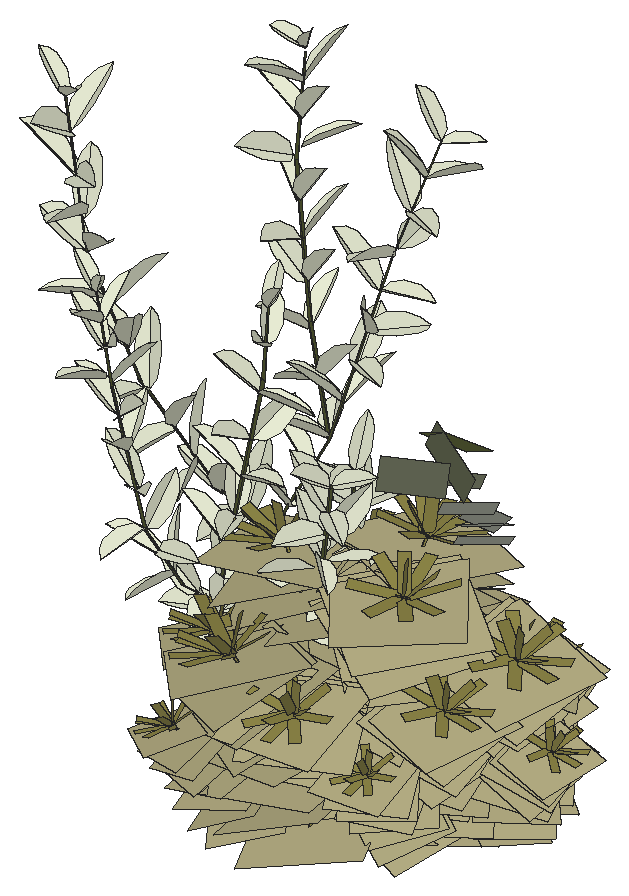
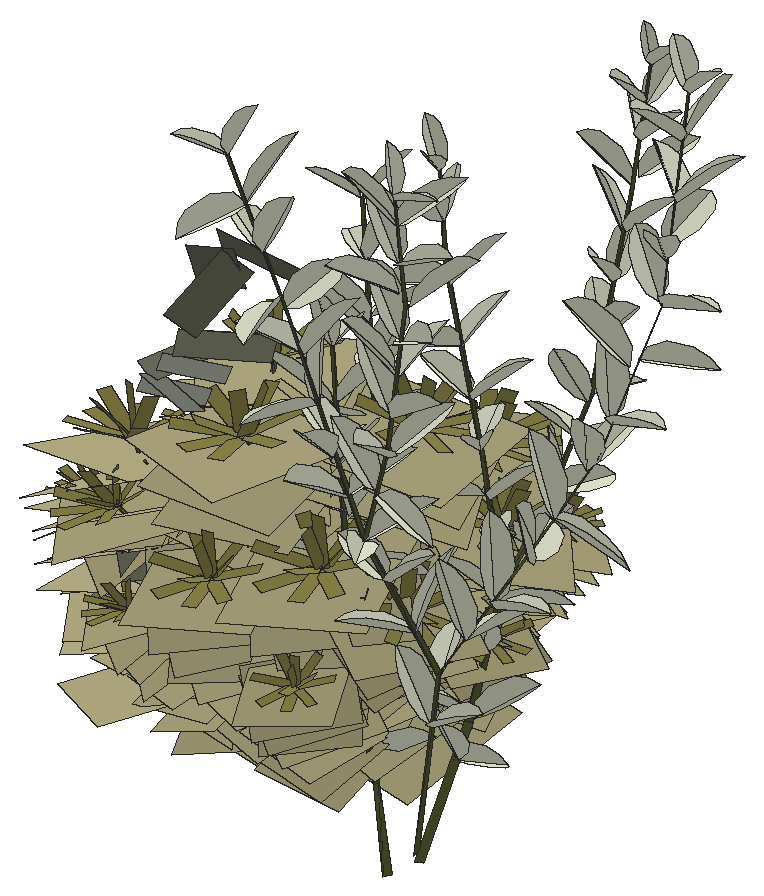
# SketchUp Ruby script. Lengths in inches.
U = 1.inch
M = Sketchup.active_model
def pt(a) = Geom::Point3d.new(a.map { |v| v * U })
def face(e, loops, mat)
  f = e.add_face(loops[0].map { |a| pt(a) })
  loops[1..].each { |l| e.add_face(l.map { |a| pt(a) }).erase! }
  f.material = f.back_material = mat if mat
  f
end
# faces: each face lists its corners as indices into pts; further lists are holes
def faces(e, pts, list, mat = nil) = list.each { |f| face(e, (f[0].is_a?(Array) ? f : [f]).map { |l| l.map { |i| pts[i] } }, mat) }
# xy, xz, yz: faces in a plane at the given z, y or x. An outline is a flat list of corners, or four numbers for a rectangle; further outlines are holes
def ring(l) = l.size == 4 ? [[l[0], l[1]], [l[2], l[1]], [l[2], l[3]], [l[0], l[3]]] : l.each_slice(2).to_a
def flat(e, list, mat, &to3) = list.each { |f| face(e, (f[0].is_a?(Array) ? f : [f]).map { |l| ring(l).map { |u, v| to3.(u, v) } }, mat) }
def xy(e, z, list, mat = nil) = flat(e, list, mat) { |x, y| [x, y, z] }
def xz(e, y, list, mat = nil) = flat(e, list, mat) { |x, z| [x, y, z] }
def yz(e, x, list, mat = nil) = flat(e, list, mat) { |y, z| [x, y, z] }
def lines(e, pts, list) = list.each { |a, b| e.add_line(pt(pts[a]), pt(pts[b])) }
# prism: a flat outline (further loops are holes) pulled along v
def prism(e, loops, v, mat = nil)
  f = face(e, loops, mat); d = Geom::Vector3d.new(v.map { |x| x * U })
  f.pushpull(f.normal.samedirection?(d) ? d.length : -d.length)
end
def box(e, o, s, mat = nil) = prism(e, [[o, [o[0] + s[0], o[1], o[2]], [o[0] + s[0], o[1] + s[1], o[2]], [o[0], o[1] + s[1], o[2]]]], [0, 0, s[2]], mat)
def at(x, y, z, deg = 0) = Geom::Transformation.translation(pt([x, y, z])) * Geom::Transformation.rotation(ORIGIN, Z_AXIS, deg.degrees)
def axes(o, x, y, z) = Geom::Transformation.new([*x, 0, *y, 0, *z, 0, *pt(o).to_a, 1])
def part(name) = M.definitions.add(name)
# library, detail: a bought-in or finely detailed component or shape, given as its bounding box
def library(name, o, s) = part(name).tap { |d| box(d.entities, o, s) }
def detail(e, o, s) = box(e.add_group.entities, o, s)
def put(e, d, t, mat = nil) = e.add_instance(d, t).tap { |i| i.material = mat if mat }
def group(e, t, mat = nil) = e.add_group.tap { |g| g.transformation = t; g.material = mat if mat }.entities
root = M.entities
M.materials.add("0ad16as01f6asdLeafVar1sfd015as60f1as6").color = [231, 235, 211]
M.materials.add("Colorsadfasdfa0sd1f06w3").color = [153, 130, 61]
M.materials.add("Euphorbia asdfasd0f150160s159w").color = [180, 173, 131]
M.materials.add("Euphorbiaasdfa0sdf1a56sd016wow Leaf SU").color = [141, 134, 72]
M.materials.add("asdfasdf0165f6asdLeafVar1sfd015as60f1as6").color = [231, 235, 211]
M.materials.add("dw_stemssadfasdfa0sdf1s01d6w1").color = [90, 97, 50]
M.materials.add("viburnumblaasdfas0df1w06d").color = [98, 102, 84]
M.materials.add("viburnumbladsadfasdfad0w122").color = [125, 129, 119]
c1 = part("vdw_leaf\#2")
p = [[0,0,0],[-2.77,1.61,2.32],[-4.3125,6.1,4.5],[-3.97,13.49,6.09],[-2.47,18.57,6.3],[-0.2,22.73,5.75],
  [2.54,19.66,6.85],[4.3,15.93,7.09],[5.03,7.6,5.43],[3.32,1.76,2.74]]
faces(c1.entities,p,[[0,1,2,3,4,5],[0,5,6,7,8,9]],"asdfasdf0165f6asdLeafVar1sfd015as60f1as6")
c2 = part("dg_branch_1\#2")
p = [[46.12,1.57,35.62],[46,5.42,35.41],[0.14,1.79,0.05],[0.26,-2.0625,0.27],[74.05,2.99,75.8],[74.11,5.28,75.58],
  [103.46,0.47,94.74],[104.03,2.92,94.84],[81.14,16.92,120.46],[81.2,18.78,120.24],[130.47,-5.6875,130.27],[130.58,-3.66,129.85],
  [80.82,34.4375,191.22],[80.64,35.93,190.9],[148.49,-14.56,203.24],[148.9,-12.8125,203.11],[81.08,37.95,226.93],[81.4,39.1,227.03],
  [157.45,-18.19,250.77],[157.7,-17.01,250.41]]
faces(c2.entities,p,[[0,1,2,3],[4,0,1],[4,1,5],[6,4,5],[6,5,7],[8,4,5],[8,5,9],[10,6,7],
  [10,7,11],[12,8,9],[12,9,13],[14,10,11],[14,11,15],[16,12,13],[16,13,17],[18,14,15],
  [18,15,19]],"dw_stemssadfasdfa0sdf1s01d6w1")
c3 = part("vdw_branch1\#3")
put(c3.entities,c1,axes([120.69,-2.42,117.31],[1.12221,-0.24063,-0.65809],[0.19207,1.24776,-0.12871],[0.65778,0.01392,1.11658]))
put(c3.entities,c1,axes([81,38.9,226.05],[0.7888,-0.58155,0],[0.48308,0.65523,0.47],[-0.28484,-0.38635,0.83138]))
put(c3.entities,c1,axes([78.08,12.69,106.05],[-1.43826,-0.02353,-0.03177],[0.0088,-1.31777,0.57755],[-0.03854,0.57714,1.31741]))
put(c3.entities,c1,axes([130.18,-4.73,130.41],[-0.38031,-1.29044,-0.11242],[1.20662,-0.31032,-0.51987],[0.47109,-0.24694,1.24081]))
put(c3.entities,c1,axes([157.08,-17.89,249.93],[-0.91355,0.40674,0],[-0.37496,-0.84216,0.38752],[0.15762,0.35401,0.92186]))
put(c3.entities,c1,axes([90.64,3.03,86.49],[0.32514,-0.85045,-0.99675],[0.69523,0.98247,-0.61148],[1.11061,-0.36604,0.67459]))
put(c3.entities,c1,axes([80.15,28.42,160.95],[-0.16039,0.95636,-1.06292],[-1.41646,0.03966,0.24943],[0.19509,1.07422,0.93709]))
put(c3.entities,c1,axes([126.74,-5.45,129.22],[-0.59819,0.96152,-0.6841],[-0.85772,0.12575,0.92675],[0.75427,0.88089,0.57856]))
put(c3.entities,c1,axes([133.22,-6.12,150.66],[-0.93823,0.76985,0.59124],[-0.47726,-1.08188,0.65135],[0.84525,0.24366,1.02405]))
put(c3.entities,c1,axes([80.43,22.89,141.32],[-1.42571,-0.19312,0.01373],[0.18338,-1.31425,0.5561],[-0.0621,0.5528,1.32692]))
put(c3.entities,c1,axes([33.14,0.88,26.42],[-0.13338,1.31536,0.04876],[-1.04528,-0.13221,0.7073],[0.72315,0.03348,1.07497]))
put(c3.entities,c1,axes([152.63,-15.08,221.76],[-1.28188,0.41945,0.0579],[-0.3638,-1.18547,0.53367],[0.21665,0.49113,1.23869]))
put(c3.entities,c1,axes([80.05,28.28,160.33],[-0.46732,-1.26661,0.40679],[1.27397,-0.40257,0.21004],[-0.07408,0.44645,1.30501]))
put(c3.entities,c1,axes([153.95,-14.8,235.875],[0.39005,1.07743,0.20605],[-0.96443,0.25296,0.50293],[0.42961,-0.3464,0.99807]))
put(c3.entities,c1,axes([80.2,24.22,141.74],[1.33062,-0.46576,0.02628],[0.44746,1.2746,-0.06608],[-0.00197,0.0722,1.37936]))
put(c3.entities,c1,axes([145.48,-12.5,188.92],[-1.32952,0.16983,0.16138],[-0.09299,-1.2361,0.53471],[0.21503,0.51548,1.22904]))
put(c3.entities,c1,axes([139.64,-9.18,171.24],[0.05682,1.30088,0.23414],[-1.13176,-0.05343,0.57151],[0.58357,-0.22963,1.13417]))
put(c3.entities,c1,axes([70.95,4.35,71.98],[-1.1081,-0.41873,0.64752],[0.33675,-1.28259,-0.25313],[0.6937,-0.04625,1.15721]))
put(c3.entities,c1,axes([59.85,4.55,56.17],[-0.26797,1.24526,0.35754],[-0.9369,-0.41634,0.74783],[0.83377,-0.10389,0.98674]))
put(c3.entities,c1,axes([33.11,3.36,25.66],[-0.57817,-1.07968,-0.5679],[1.11554,-0.21356,-0.7297],[0.49375,-0.78178,0.98363]))
put(c3.entities,c2,at(-0.21,0.34,-0.17),"dw_stemssadfasdfa0sdf1s01d6w1")
put(c3.entities,c1,axes([80.91,19.01,122.53],[-0.84258,1.13222,-0.27981],[-1.15093,-0.75138,0.42537],[0.18861,0.47293,1.3457]))
put(c3.entities,c1,axes([119.8,-1.22,114.1],[-1.3235,-0.25012,0.09101],[0.25933,-1.31572,0.15537],[0.05991,0.1698,1.33794]))
put(c3.entities,c1,axes([46.29,5.1,38.04],[0.98937,0.73827,-0.47585],[-0.72359,1.03721,0.10473],[0.44068,0.18581,1.20453]))
put(c3.entities,c1,axes([81.1875,33.03,184.45],[1.33883,0.26986,0.35053],[-0.09581,1.22087,-0.57399],[-0.42216,0.53228,1.20262]))
put(c3.entities,c1,axes([80.16,36.28,206.98],[-0.83993,0.85737,-0.6234],[-1.05964,-0.65701,0.5241],[0.02941,0.81391,1.07976]))
put(c3.entities,c1,axes([154.86,-16.15,234.87],[0.02509,-1.15302,-0.28506],[1.1487,-0.04894,0.29908],[-0.30202,-0.28195,1.11384]))
put(c3.entities,c1,axes([108.77,-0.33,101.14],[-0.47691,-1.03266,-0.72709],[1.25395,-0.29455,-0.40416],[0.15052,-0.81814,1.06325]))
put(c3.entities,c1,axes([89.79,3.01,85.87],[-0.61344,0.75518,0.8965],[-0.17758,-1.01824,0.73622],[1.13385,0.22574,0.58569]))
put(c3.entities,c1,axes([81.56,20.31,123.29],[0.37259,-1.3435,0.21057],[1.29385,0.32364,-0.22445],[0.16906,0.25791,1.34638]))
put(c3.entities,c1,axes([46.45,1.82,36.74],[-0.77883,0.29892,1.0614],[0.19124,-1.24314,0.49044],[1.08598,0.43329,0.67484]))
put(c3.entities,c1,axes([71.37,4.02,72.32],[0.72905,0.81546,-0.74421],[-0.66805,0.98958,0.42988],[0.8391,0.14186,0.97745]))
put(c3.entities,c1,axes([136.59,-5.88,150.53],[0.85845,-0.99897,-0.12437],[0.96526,0.81273,0.13453],[-0.02572,-0.18182,1.28292]))
put(c3.entities,c1,axes([80.375,38.8,225.86],[-0.25178,0.96778,0],[-0.89216,-0.23211,0.38752],[0.37503,0.09757,0.92186]))
put(c3.entities,c1,axes([74.43,7.99,85.38],[-1.05703,0.91669,-0.33543],[-0.95806,-0.87958,0.61531],[0.18697,0.6754,1.25659]))
put(c3.entities,c1,axes([76.57,9.74,89.32],[0.63146,-1.21538,0.33508],[1.18148,0.49387,-0.43517],[0.26321,0.48577,1.26593]))
put(c3.entities,c1,axes([81.6875,36.97,207.4],[0.09422,-1.04424,0.38486],[1.01646,0.1939,0.27727],[-0.33299,0.33382,0.98727]))
put(c3.entities,c1,axes([157.29,-17.17,249.98],[0.50586,-0.50586,0],[0.38853,0.38853,0.41105],[-0.29684,-0.29684,0.56115]))
put(c3.entities,c1,axes([79.92,15.8,106.09],[1.03917,-0.29343,-0.90675],[-0.14587,1.22131,-0.5624],[0.92163,0.5191,0.88824]))
put(c3.entities,c1,axes([61.95,3.88,56.26],[0.41243,-1.28546,0],[1.17466,0.37688,-0.54831],[0.5221,0.16751,1.23363]))
put(c3.entities,c1,axes([151.99,-14.79,208.15],[-0.48571,-1.21723,-0.32393],[1.25386,-0.50033,0],[-0.12005,-0.30087,1.31056]))
put(c3.entities,c1,axes([108.44,0.62,102.22],[0.82183,0.96078,0.38967],[-0.62327,0.08618,1.10203],[0.79141,-0.88661,0.51693]))
put(c3.entities,c1,axes([145.6,-10.56,188.62],[1.03241,-0.02554,-0.82693],[0.3944,1.11584,0.45794],[0.70325,-0.61672,0.89706]))
put(c3.entities,c1,axes([78.59,32.3,183.89],[-1.12675,-0.42036,0.43987],[0.5899,-0.98149,0.57312],[0.14901,0.70693,1.05726]))
put(c3.entities,c1,axes([152.08,-13.42,223.37],[0.79993,-0.44251,-0.69938],[0.68456,0.82615,0.26026],[0.41048,-0.60953,0.85515]))
put(c3.entities,c1,axes([140.71,-8.74,170.55],[0.41903,-1.24177,-0.32393],[1.26224,0.33728,0.33986],[-0.23168,-0.40836,1.26573]))
put(c3.entities,c1,axes([149.25,-12.53,205.78],[1.24456,0.38285,0.23414],[-0.42999,1.04826,0.57151],[-0.02056,-0.62679,1.13417]))
c4 = part("Component\#314")
p = [[0.14,0,0],[2.58,0.05,0.25],[2.44,5.11,2.64],[0,5.05,2.39]]
faces(c4.entities,p,[[0,1,2,3]],"viburnumblaasdfas0df1w06d")
c5 = part("viburnumblad1\#2")
put(c5.entities,c4,axes([-37.25,6.23,19.31],[75.98784,0,0],[0,65.50676,0],[0,0,75.98784]))
c6 = part("Component\#306")
p = [[4.55,0.11,0],[4.55,0,0],[2.84,0,3.13],[2.84,0.11,3.13],[4.625,0.05,0.04],[2.92,0.05,3.15],
  [2.08,0,8.07],[2.08,0.11,8.07],[2.16,0.05,8.1],[0,0,12.54],[0,0.11,12.54],[0.07,0.05,12.58]]
faces(c6.entities,p,[[0,1,2,3],[1,4,5,2],[1,0,4],[4,0,3,5],[3,2,6,7],[2,5,8,6],[5,3,7,8],[7,6,9,10],
  [6,8,11,9],[8,7,10,11],[10,9,11]],"Colorsadfasdfa0sd1f06w3")
c7 = part("Component\#301")
xy(c7.entities,0,[[0,0,0.7,3.1]],"Euphorbiaasdfa0sdf1a56sd016wow Leaf SU")
c8 = part("Leaf rosette")
put(c8.entities,c7,axes([2.21,1.74,0.13],[-0.4441,0.47879,-0.0956],[-0.4878,-0.4406,0.05935],[-0.03146,0.16757,0.98536]))
put(c8.entities,c7,axes([2.29,1.9,0.17],[-0.62678,-0.10063,-0.18061],[0.01105,-0.59203,0.2915],[-0.31282,0.41486,0.85442]))
put(c8.entities,c7,axes([2.09,1.69,0.1],[-0.10438,0.65169,0],[-0.65169,-0.10438,0],[0,0,1]))
put(c8.entities,c7,axes([1.97,1.77,0.02],[0.31114,0.5228,0.25587],[-0.57125,0.32993,0.02052],[-0.16918,-0.3502,0.92127]))
put(c8.entities,c7,axes([1.93,1.95,0],[0.54816,-0.03215,0.36617],[-0.11878,0.60671,0.23108],[-0.52706,-0.39065,0.75472]))
put(c8.entities,c7,axes([2.04,2.1,0.05],[0.26275,-0.55867,0.23335],[0.34186,0.34684,0.44545],[-0.75711,-0.08556,0.64766]))
put(c8.entities,c7,axes([2.22,2.08,0.13],[-0.29265,-0.59104,-0.02512],[0.40323,-0.2198,0.47401],[-0.65583,0.2952,0.69479]))
c9 = part("Component\#308")
xy(c9.entities,0,[[0,0,5.01,4.64]],"Euphorbia asdfasd0f150160s159w")
c10 = part("Component\#316")
put(c10.entities,c6,at(2.35,3.5,0))
put(c10.entities,c8,at(0.25,1.59,12.45))
put(c10.entities,c9,axes([7.46,0.77,3.64],[0.10848,0.99337,0.03799],[-0.82378,0.11122,-0.55589],[-0.55643,0.02901,0.83038]))
put(c10.entities,c9,axes([1.97,2.58,1.93],[0.80762,-0.50565,0.30344],[0.47433,0.86274,0.17519],[-0.35038,0.00244,0.93661]))
put(c10.entities,c9,axes([5.79,0.14,3.9],[0.5013,0.78918,0.35482],[-0.74775,0.60146,-0.2813],[-0.4354,-0.1243,0.89162]))
put(c10.entities,c9,axes([1.87,2.6,3.75],[0.73154,-0.49698,0.46676],[0.47433,0.86274,0.17519],[-0.48976,0.09324,0.86686]))
put(c10.entities,c9,axes([3.91,7.06,6.66],[-0.50827,-0.83837,-0.19699],[0.8278,-0.53869,0.15675],[-0.23753,-0.08339,0.96779]))
put(c10.entities,c9,axes([1.2,3.99,6.83],[0.56066,-0.79708,0.22433],[0.74237,0.60386,0.29025],[-0.36682,0.0038,0.93028]))
put(c10.entities,c7,axes([2.42,3.73,12.57],[-0.1322,-0.64472,0.04955],[0.10064,0.02944,0.65162],[-0.9678,0.2092,0.14002]))
put(c10.entities,c7,axes([2.57,3.43,12.63],[-0.62833,0.089,-0.18134],[-0.19954,-0.36568,0.51192],[-0.04764,0.82148,0.56824]))
put(c10.entities,c9,axes([4.04,6.92,11.09],[-0.67411,-0.5063,-0.5378],[0.44628,-0.85937,0.24964],[-0.58857,-0.07172,0.80526]))
put(c10.entities,c7,axes([2.5,3.49,12.74],[-0.62833,0.089,-0.18134],[-0.18746,-0.03618,0.63178],[0.11402,0.98935,0.09049]))
put(c10.entities,c7,axes([2.3,3.27,12.51],[0.02916,0.64747,0.12464],[-0.56235,-0.04072,0.34308],[0.5216,-0.18387,0.83314]))
put(c10.entities,c9,axes([0.26,4.96,9.69],[0.33661,-0.92735,0.16343],[0.73504,0.36725,0.56995],[-0.58857,-0.07172,0.80526]))
put(c10.entities,c9,axes([4.76,6.31,12.62],[-0.95056,-0.1129,-0.28929],[0.09021,-0.99179,0.09066],[-0.29715,0.06008,0.95294]))
put(c10.entities,c9,axes([5.2,6.55,10.37],[-0.76372,-0.27738,-0.58291],[0.26517,-0.95808,0.10848],[-0.58857,-0.07172,0.80526]))
c11 = part("Plant stem")
p = [[2.84,0.11,3.13],[2.84,0,3.13],[2.08,0,8.07],[2.08,0.11,8.07],[2.92,0.05,3.15],[2.16,0.05,8.1],
  [0,0,12.54],[0,0.11,12.54],[0.07,0.05,12.58]]
faces(c11.entities,p,[[0,1,2,3],[1,4,5,2],[4,0,3,5],[3,2,6,7],[2,5,8,6],[5,3,7,8],[7,6,8]],"Colorsadfasdfa0sd1f06w3")
c12 = part("Leafy shoot")
put(c12.entities,c11,at(2.35,3.5,0))
put(c12.entities,c8,at(0.25,1.59,12.45))
put(c12.entities,c9,axes([1.87,2.6,3.75],[0.73154,-0.49698,0.46676],[0.47433,0.86274,0.17519],[-0.48976,0.09324,0.86686]))
put(c12.entities,c9,axes([3.91,7.06,6.66],[-0.50827,-0.83837,-0.19699],[0.8278,-0.53869,0.15675],[-0.23753,-0.08339,0.96779]))
put(c12.entities,c9,axes([1.2,3.99,6.83],[0.56066,-0.79708,0.22433],[0.74237,0.60386,0.29025],[-0.36682,0.0038,0.93028]))
put(c12.entities,c7,axes([2.42,3.73,12.57],[-0.1322,-0.64472,0.04955],[0.10064,0.02944,0.65162],[-0.9678,0.2092,0.14002]))
put(c12.entities,c7,axes([2.57,3.43,12.63],[-0.62833,0.089,-0.18134],[-0.19954,-0.36568,0.51192],[-0.04764,0.82148,0.56824]))
put(c12.entities,c9,axes([4.04,6.92,11.09],[-0.67411,-0.5063,-0.5378],[0.44628,-0.85937,0.24964],[-0.58857,-0.07172,0.80526]))
put(c12.entities,c7,axes([2.5,3.49,12.74],[-0.62833,0.089,-0.18134],[-0.18746,-0.03618,0.63178],[0.11402,0.98935,0.09049]))
put(c12.entities,c7,axes([2.3,3.27,12.51],[0.02916,0.64747,0.12464],[-0.56235,-0.04072,0.34308],[0.5216,-0.18387,0.83314]))
put(c12.entities,c9,axes([0.26,4.96,9.69],[0.33661,-0.92735,0.16343],[0.73504,0.36725,0.56995],[-0.58857,-0.07172,0.80526]))
put(c12.entities,c9,axes([4.76,6.31,12.62],[-0.95056,-0.1129,-0.28929],[0.09021,-0.99179,0.09066],[-0.29715,0.06008,0.95294]))
put(c12.entities,c9,axes([5.2,6.55,10.37],[-0.76372,-0.27738,-0.58291],[0.26517,-0.95808,0.10848],[-0.58857,-0.07172,0.80526]))
put(c12.entities,c9,axes([7.03,0.77,3.77],[0.19714,0.84663,0.32426],[-0.94994,0.28899,-0.30484],[-0.2731,-0.45173,0.91532]))
c13 = part("Groundcover plant")
put(c13.entities,c10,axes([0.82,1.83,0.8125],[0.98541,0,-0.17021],[0,1,0],[0.17021,0,0.98541]))
put(c13.entities,c12,axes([4.45,-0.84,-2.24],[0.69527,0.50616,0],[-0.50264,0.69042,-0.10135],[-0.05965,0.08194,0.85401]))
put(c13.entities,c12,axes([1.85,7.37,-3.38],[0.7038,-0.47341,0.14191],[0.46407,0.71797,0.09357],[-0.16999,0,0.84303]))
put(c13.entities,c12,axes([6.9,-3.65,-2.52],[0.79351,0.57769,0],[-0.57366,0.78798,-0.11567],[-0.06808,0.09351,0.97468]))
put(c13.entities,c12,axes([1.36,5.18,-2.66],[0.50674,-0.34086,0.10218],[0.33413,0.51694,0.06737],[-0.12239,0,0.60698]))
put(c13.entities,c12,axes([5.76,-1.49,-2.17],[0.43479,0.43181,0.07251],[-0.43488,0.43544,-0.06951],[-0.06212,-0.06169,0.61918]))
c14 = part("Groundcover clump")
put(c14.entities,c13,axes([25.06,6.72,0.82],[-0.74291,1.22188,0],[-1.22188,-0.74291,0],[0,0,1]))
put(c14.entities,c13,axes([-0.76,2.1875,0.82],[1.43,0,0],[0,1.43,0],[0,0,1]))
put(c14.entities,c13,axes([8.21,24.79,0.82],[-0.6403,-1.27864,0],[1.27864,-0.6403,0],[0,0,1]))
c15 = part("vdw_leaf\#3")
p = [[0,0,0],[-2.77,1.61,2.32],[-4.3125,6.1,4.5],[-3.97,13.49,6.09],[-2.47,18.57,6.3],[-0.2,22.73,5.75],
  [2.54,19.66,6.85],[4.3,15.93,7.09],[5.03,7.6,5.43],[3.32,1.76,2.74]]
faces(c15.entities,p,[[0,1,2,3,4,5],[0,5,6,7,8,9]],"asdfasdf0165f6asdLeafVar1sfd015as60f1as6")
c16 = part("dw_brancj_2\#2")
p = [[9.7,-0.22,29.95],[0.23,-1.96,0.34],[-0.05,1.51,0.11],[9.65,1.51,29.46],[18.64,-8.75,84.43],[18.96,-6.63,84.625],
  [1.53,6.02,63.68],[1.42,8.18,63.25],[-10.58,8.77,161.17],[-10.41,9.98,160.68],[26.34,-9.37,211.72],[26.57,-8.28,211.23]]
faces(c16.entities,p,[[0,1,2],[0,2,3],[4,0,3],[4,3,5],[6,0,3],[6,3,7],[8,6,7],[8,7,9],
  [10,4,5],[10,5,11]],"dw_stemssadfasdfa0sdf1s01d6w1")
c17 = part("vdw_branch2\#3")
put(c17.entities,c15,axes([19.53,-5.9,102.42],[1.12377,-0.50004,0],[0.46097,1.03596,0.47664],[-0.19377,-0.43548,1.13389]))
put(c17.entities,c15,axes([-5.89,6.52,109.44],[-1.07209,0.83679,0],[-0.77141,-0.98832,0.52702],[0.32427,0.41545,1.25373]))
put(c17.entities,c15,axes([-0.44,8.23,75.28],[0.88709,-0.9947,0],[0.92159,0.82189,0.33087],[-0.25219,-0.22491,1.26111]))
put(c17.entities,c15,axes([24.71,-8.97,190.81],[-0.82641,0.91101,0],[-0.83983,-0.76184,0.47664],[0.35303,0.32025,1.13389]))
put(c17.entities,c15,axes([-2.29,8.24,91.35],[1.24603,-0.47303,0],[0.43826,1.15445,0.33087],[-0.11993,-0.31592,1.26111]))
put(c17.entities,c15,axes([12.26,-3.11,37.92],[-0.64625,1.02205,0.22511],[-1.04383,-0.61044,-0.22511],[-0.07533,-0.30931,1.18809]))
put(c17.entities,c15,axes([26.17,-9.17,210.27],[-0.99452,-0.10453,0],[0.09636,-0.91681,0.38752],[-0.04051,0.38539,0.92186]))
put(c17.entities,c15,axes([-6.07,9.4,125.35],[-0.90214,-0.98107,0],[0.90896,-0.83583,0.33087],[-0.24874,0.22873,1.26111]))
put(c17.entities,c15,axes([-4.13,7.29,110.58],[0.44715,-1.078,0.64369],[1.05816,0.63649,0.33087],[-0.58725,0.40856,1.09216]))
put(c17.entities,c15,axes([23.91,-8.22,171.96],[0.62307,0.85009,-0.63406],[-0.71531,0.8798,0.47664],[0.78296,0.12729,0.94004]))
put(c17.entities,c16,at(-0.09,0.18,-0.25),"dw_stemssadfasdfa0sdf1s01d6w1")
put(c17.entities,c15,axes([23.34,-9.65,156.59],[-0.31364,-1.00782,0.58216],[1.10369,-0.17062,0.29925],[-0.17137,0.6239,0.98776]))
put(c17.entities,c15,axes([15.03,-3.37,58.83],[-1.05425,-0.00194,0.58442],[-0.14303,-1.11707,-0.26172],[0.55355,-0.3046,0.99755]))
put(c17.entities,c15,axes([-11.625,9.46,160.37],[0.36812,0.92978,0],[-0.85713,0.33936,0.38752],[0.3603,-0.14265,0.92186]))
put(c17.entities,c15,axes([21.32,-8.53,138.72],[1.21379,0.19904,0],[-0.19904,1.21379,0],[0,0,1.23]))
put(c17.entities,c15,axes([22.54,-9.2,141.43],[-1.02887,0.17955,0.60182],[-0.23387,-1.13057,-0.06253],[0.56696,-0.17376,1.02111]))
put(c17.entities,c15,axes([23.9,-8.82,173.84],[-1.14567,-0.37474,0],[0.35918,-1.0981,0.04438],[-0.01409,0.04308,1.17993]))
put(c17.entities,c15,axes([-7.84,8.92,143.59],[-1.26971,0.40522,0],[-0.37543,-1.17638,0.33087],[0.10274,0.32192,1.26111]))
put(c17.entities,c15,axes([19.77,-8.01,85.98],[-0.32405,-1.14591,0.18674],[1.10278,-0.32969,-0.10948],[0.15845,0.14442,1.16117]))
put(c17.entities,c15,axes([-0.62,5.76,76.34],[-0.08879,1.17576,-0.67771],[-1.34525,-0.16582,-0.11144],[-0.17897,0.66309,1.17383]))
put(c17.entities,c15,axes([20.49,-8.22,121.07],[0.39924,-0.78471,-0.8233],[1.08735,0.33121,0.2116],[0.09035,-0.83005,0.83495]))
put(c17.entities,c15,axes([15.15,-3.72,62.9],[1.16251,0.40128,-0.0211],[-0.39924,1.16074,0.07874],[0.0456,-0.06757,1.2273]))
put(c17.entities,c15,axes([20.72,-8.08,120.26],[-0.03693,1.2277,-0.06551],[-1.22944,-0.03698,0],[-0.00197,0.06548,1.22825]))
put(c17.entities,c15,axes([22.58,-8.36,155.57],[-0.56247,1.09386,0],[-1.00839,-0.51852,0.47664],[0.42389,0.21796,1.13389]))
put(c17.entities,c15,axes([3.97,3.13,57.96],[-1.09459,0.76041,0],[-0.72262,-1.0402,-0.1735],[-0.10109,-0.14552,1.29352]))
put(c17.entities,c15,axes([-10.8,9.06,160.75],[-0.66334,-0.72138,0],[0.66835,-0.61458,0.24329],[-0.1829,0.16818,0.92729]))
put(c17.entities,c15,axes([19.06,-9.3125,103.96],[-1.01345,0.25553,-0.60051],[-0.2265,-1.12952,-0.09839],[-0.59598,0.03076,1.01889]))
put(c17.entities,c15,axes([18.07,-6.2,81.7],[-0.56247,1.09386,0],[-1.00839,-0.51852,0.47664],[0.42389,0.21796,1.13389]))
put(c17.entities,c15,axes([12.95,-0.39,43.31],[0.13044,-1.19832,0],[1.11025,0.12085,0.29925],[-0.30382,-0.03307,1.14057]))
put(c17.entities,c15,axes([2.28,8.28,56.18],[1.32413,-0.31027,0],[0.30923,1.31968,-0.11144],[0.02542,0.1085,1.35543]))
put(c17.entities,c15,axes([-7.55,9.96,143.07],[1.34251,-0.21744,0],[0.20045,1.23761,0.52702],[-0.08426,-0.52024,1.25373]))
put(c17.entities,c15,axes([26.15,-8.25,210.66],[0.94661,-0.25364,0],[0.235,0.87703,0.24329],[-0.06431,-0.24,0.92729]))
put(c17.entities,c15,axes([-6.48,11.37,125.16],[0.64635,1.10315,0.46356],[-1.16569,0.46153,0.52702],[0.27017,-0.6478,1.16488]))
put(c17.entities,c15,axes([25.74,-8.35,191.28],[0.13044,-1.19832,0],[1.11025,0.12085,0.29925],[-0.30382,-0.03307,1.14057]))
put(c17.entities,c15,axes([-5.125,7.47,91.6],[-1.10024,0.63688,0.48318],[-0.78682,-1.00808,-0.46292],[0.14137,-0.65404,1.184]))
c18 = part("Component\#315")
p = [[0.25,0,0],[2.05,0.01,0.35],[1.81,4.2,1.66],[0,4.19,1.3125]]
faces(c18.entities,p,[[0,1,2,3]],"viburnumbladsadfasdfad0w122")
c19 = part("viburnumblad2")
put(c19.entities,c18,axes([-19.23,-4.49,-32.18],[83.35428,0,0],[0,79.38502,0],[0,0,83.35428]))
c20 = part("vdw_leaf\#1")
p = [[0,0,0],[-2.77,1.61,2.32],[-4.3125,6.1,4.5],[-3.97,13.49,6.09],[-2.47,18.57,6.3],[-0.2,22.73,5.75],
  [2.54,19.66,6.85],[4.3,15.93,7.09],[5.03,7.6,5.43],[3.32,1.76,2.74]]
faces(c20.entities,p,[[0,1,2,3,4,5],[0,5,6,7,8,9]],"0ad16as01f6asdLeafVar1sfd015as60f1as6")
c21 = part("dw_branch_3\#2")
p = [[-10.06,-1.6,62.9],[-0.2,1.54,-0.01],[-10.43,1.54,62.72],[0.18,-1.6,0.17],[-23.75,-21.66,88.91],[-25.7,-20.3,89.55],
  [13.4,11.62,104.56],[13.33,13.52,104.47],[-49.25,-41.87,130.3125],[-50.33,-40.21,130.71],[-4.97,21.13,143.98],[35.61,27.99,178.64],
  [-5.09,23.64,143.96],[35.32,29.14,178.46],[-67.7,-55.38,181.06],[-68.34,-54.45,181.62],[-22.8125,33.9,200.59],[-22.94,35.79,200.41],
  [56.61,36.78,229.75],[56.29,38.09,229.57],[-70.63,-67.46,248.85],[-70.72,-66.33,249.5],[-25.05,43.32,240.75],[-24.98,44.26,240.57]]
faces(c21.entities,p,[[0,1,2],[0,3,1],[4,2,5],[4,0,2],[6,0,2],[6,2,7],[8,4,5],[8,5,9],
  [10,6,7],[11,6,7],[10,7,12],[11,7,13],[14,8,9],[14,9,15],[16,10,12],[16,12,17],
  [18,11,13],[18,13,19],[20,14,15],[20,15,21],[22,16,17],[22,17,23]],"dw_stemssadfasdfa0sdf1s01d6w1")
c22 = part("dw_branch3\#2")
put(c22.entities,c20,axes([-70.33,-63.58,233.32],[-1.00752,0.412,0.78596],[-0.24851,-1.22189,0.32195],[0.83141,0.09817,1.01433]))
put(c22.entities,c20,axes([-66.93,-54.91,182.82],[-0.84976,-0.98359,0.33619],[0.99572,-0.74889,0.32577],[-0.05223,0.46521,1.22907]))
put(c22.entities,c20,axes([-46.12,-39.49,126.35],[1.23843,0.5364,0.23552],[-0.56438,0.94474,0.81599],[0.15707,-0.83465,1.07498]))
put(c22.entities,c20,axes([13.0625,13.13,104.77],[-1.01271,0.69982,-0.26884],[-0.74268,-0.99813,0.19939],[-0.10222,0.31872,1.21473]))
put(c22.entities,c20,axes([-18.87,30.42,186.42],[0.36309,1.06515,-0.56675],[-1.14134,0.49515,0.19939],[0.39128,0.45593,1.10754]))
put(c22.entities,c20,axes([-3.2,4.15,75.77],[-1.04153,0.55414,0.44243],[-0.23365,-1.01045,0.71554],[0.6695,0.50943,0.93801]))
put(c22.entities,c20,axes([23.2,19.41,136.3],[-0.65687,-1.11295,-0.05714],[1.05857,-0.61429,-0.20411],[0.15163,-0.1536,1.24868]))
put(c22.entities,c20,axes([-25.57,35.48,201.32],[-0.64726,0.62827,0.87973],[-0.71635,-1.0172,0.19939],[0.80962,-0.39773,0.87973]))
put(c22.entities,c20,axes([-36.37,-32.14,110.35],[-0.80747,1.09962,0.12544],[-0.83333,-0.50188,-0.96467],[-0.72833,-0.64487,0.96467]))
put(c22.entities,c20,axes([-9.89,26.72,156.79],[0.45529,1.02969,0.56572],[-1.16919,0.33753,0.32662],[0.11537,-0.64297,1.07744]))
put(c22.entities,c20,axes([-26.57,46.1,241.0625],[0.00015,0.80921,0.22536],[-0.83985,0.00446,-0.01542],[-0.01605,-0.22532,0.80906]))
put(c22.entities,c20,axes([-9.2,-2.58,61.06],[-1.10001,-0.40312,0.39014],[0.40883,-1.1116,0.00411],[0.35732,0.13566,1.14763]))
put(c22.entities,c20,axes([-69.91,-63.11,233.93],[1.36249,-0.1432,0],[0.13201,1.25603,0.5309],[-0.05549,-0.52799,1.26295]))
put(c22.entities,c20,axes([32.2,25.46,166.13],[0.06878,-1.29051,-0.05714],[1.22165,0.07415,-0.20411],[0.2113,-0.04403,1.24868]))
put(c22.entities,c20,axes([-5.68,-0.66,44.43],[-0.48448,-1.12287,0.17078],[0.98138,-0.33653,0.57135],[-0.48308,0.36756,1.04626]))
put(c22.entities,c20,axes([43.45,32.81,198.64],[0.5408,1.19584,0.14106],[-0.94242,0.32409,0.86557],[0.74952,-0.45533,0.98656]))
put(c22.entities,c20,axes([12.52,14.14,104.98],[1.02694,0.54888,0.41092],[-0.53566,1.05407,-0.06927],[-0.38969,-0.12321,1.13846]))
put(c22.entities,c20,axes([44.55,32.375,198.73],[-0.65687,-1.11295,-0.05714],[1.05857,-0.61429,-0.20411],[0.15163,-0.1536,1.24868]))
put(c22.entities,c20,axes([-5.67,21.17,141.44],[-1.10726,0.43603,-0.32953],[-0.49537,-1.03435,0.29588],[-0.17521,0.40597,1.12589]))
put(c22.entities,c20,axes([55.69,37.84,229.48],[0.18984,0.96334,0.18958],[-0.71996,0.0053,0.69399],[0.66755,-0.26823,0.69457]))
put(c22.entities,c20,axes([-21.52,36.85,205.2],[0.72606,-0.98817,0.14519],[0.94364,0.7084,0.10251],[-0.16885,0.05176,1.19664]))
put(c22.entities,c20,axes([-68.51,-56.35,196.07],[1.16319,0.72381,0],[-0.66725,1.0723,0.5309],[0.28049,-0.45075,1.26295]))
put(c22.entities,c21,at(0.01,-0.09,-0.02),"dw_stemssadfasdfa0sdf1s01d6w1")
put(c22.entities,c20,axes([-2.49,5.18,75.91],[0.78614,-0.90346,-0.30078],[0.86953,0.79562,-0.11715],[0.28546,-0.14014,1.16705]))
put(c22.entities,c20,axes([-23.125,-16.22,82.25],[0.32175,1.32576,0.12544],[-1.33153,0.31835,0.05068],[0.01989,-0.13382,1.3633]))
put(c22.entities,c20,axes([-23.75,41.99,230.3],[0.85958,-0.87451,0.14519],[0.66531,0.75721,0.62192],[-0.54076,-0.36226,1.01955]))
put(c22.entities,c20,axes([27.07,22.48,149.34],[0.92952,-0.64745,-0.62467],[0.50188,1.074,-0.36637],[0.71693,0.02135,1.04468]))
put(c22.entities,c20,axes([17.66,16.25,119.93],[-0.91649,0.83891,-0.3601],[-0.87434,-0.77966,0.40896],[0.0492,0.54447,1.14321]))
put(c22.entities,c20,axes([-68.37,-54.54,181.63],[0.32047,1.28399,0.35434],[-1.33153,0.31835,0.05068],[-0.03484,-0.35624,1.32241]))
put(c22.entities,c20,axes([-28.98,-27.1,96.48],[-0.8814,-0.35966,-0.98523],[0.75246,-1.11336,-0.26672],[-0.73065,-0.71272,0.91382]))
put(c22.entities,c20,axes([-15.23,28.43,172.72],[-1.21149,0.11898,0.32517],[-0.09739,-1.25259,0.09551],[0.33228,0.0667,1.21356]))
put(c22.entities,c20,axes([-17.5625,31.23,186.85],[-0.49275,-1.12287,0.14519],[0.95014,-0.33653,0.62192],[-0.53717,0.36756,1.01955]))
put(c22.entities,c20,axes([26.7,21.22,149.39],[-1.00104,0.22334,0.83093],[0.36894,-1.0402,0.72406],[0.77731,0.78134,0.72643]))
put(c22.entities,c20,axes([-31.125,-24.87,97.38],[0.75482,-0.86936,0.69068],[-0.00159,0.80023,1.00899],[-1.08766,-0.58016,0.45842]))
put(c22.entities,c20,axes([-71.21,-66.73,248.67],[0.25207,0.96771,0],[-0.8921,0.23237,0.38752],[0.375,-0.09768,0.92186]))
put(c22.entities,c20,axes([-24.11,41.05,229.55],[-1.11612,0.51924,-0.26884],[-0.56394,-1.10897,0.19939],[-0.15444,0.29694,1.21473]))
put(c22.entities,c20,axes([6.75,8.37,91.63],[-0.33418,-1.12287,0.39014],[1.13558,-0.33653,0.00411],[0.10478,0.36756,1.14763]))
put(c22.entities,c20,axes([-26,45.89,241.63],[-0.26986,-0.70824,-0.32129],[0.56818,-0.39091,0.38449],[-0.49365,-0.09775,0.63011]))
put(c22.entities,c20,axes([3.74,17.32,124.35],[0.22441,1.22913,-0.16274],[-1.07812,0.11178,-0.64246],[-0.61228,0.25367,1.07162]))
put(c22.entities,c20,axes([-5.44,22.27,140.88],[1.2203,0.00475,0.31374],[-0.097,1.20386,0.35905],[-0.29841,-0.37189,1.1663]))
put(c22.entities,c20,axes([-13.79,29.35,173.31],[0.83169,-0.90108,0.14519],[0.68877,0.73594,0.62192],[-0.55187,-0.34509,1.01955]))
put(c22.entities,c20,axes([-16.92,-7.26,72.98],[1.30647,0.30378,-0.27886],[0.07026,0.74892,1.14503],[0.40633,-1.10623,0.69861]))
put(c22.entities,c20,axes([4.8,17.55,125.22],[-0.25598,-1.17842,0.26559],[1.01553,-0.08455,0.60363],[-0.56975,0.35087,1.00767]))
put(c22.entities,c20,axes([5.3125,8.35,91.45],[0.00638,1.22913,-0.27714],[-1.16413,0.11178,0.46895],[0.48205,0.25367,1.13617]))
put(c22.entities,c20,axes([38.12,30.57,183.07],[1.12534,0.26182,-0.63833],[-0.46674,1.18829,-0.33545],[0.5081,0.51169,1.10563]))
put(c22.entities,c20,axes([-70.41,-60.38,214.47],[-0.41425,1.30587,0],[-1.20383,-0.38188,0.5309],[0.50605,0.16053,1.26295]))
put(c22.entities,c20,axes([37.03,28.75,180.67],[-1.12533,0.00102,-0.63799],[-0.00113,-1.2408,0],[-0.62497,0.00057,1.10237]))
put(c22.entities,c20,axes([30.71,25.35,165.96],[-0.1364,1.29314,0.22715],[-1.08768,-0.23921,0.70862],[0.73536,-0.11394,1.09026]))
put(c22.entities,c20,axes([-38.05,-30.84,110.67],[-0.31533,-1.27379,-0.2839],[1.018,-0.40311,0.67794],[-0.74394,-0.05723,1.08307]))
put(c22.entities,c20,axes([50.11,34.45,213.36],[-1.05669,0.74401,-0.05714],[-0.616,-0.82138,0.69675],[0.37221,0.60904,1.04705]))
put(c22.entities,c20,axes([-65.32,-58.78,200.07],[-1.14597,-0.19668,-0.6713],[0.21784,-1.26924,0],[-0.64812,-0.11124,1.139]))
put(c22.entities,c20,axes([-53.2,-43.37,143.59],[-0.72817,-1.09167,-0.2839],[0.82127,-0.72411,0.67794],[-0.71934,0.19815,1.08307]))
put(c22.entities,c20,axes([-61.1,-50.25,163.67],[-0.52887,1.19686,-0.30066],[-1.10762,-0.57104,-0.32484],[-0.42634,0.12264,1.23812]))
put(c22.entities,c20,axes([-54.12,-42.96,142.67],[0.32175,1.32576,0.12544],[-1.33153,0.31835,0.05068],[0.01989,-0.13382,1.3633]))
put(c22.entities,c20,axes([22.03,20.08,132.3],[1.17066,0.5058,-0.34078],[-0.35758,1.16671,0.50333],[0.49407,-0.35407,1.17172]))
put(c22.entities,c20,axes([-8.59,26.04,158.21],[-0.49275,-1.12287,0.14519],[0.95014,-0.33653,0.62192],[-0.53717,0.36756,1.01955]))
put(c22.entities,c20,axes([49.92,34.03,213.7],[1.24742,-0.35176,0.25024],[0.42127,1.159,-0.4708],[-0.09426,0.52477,1.20753]))
put(c22.entities,c20,axes([-70.34,-67.02,249.05],[-0.57048,-0.79684,0],[0.73827,-0.52855,0.24329],[-0.20203,0.14464,0.92729]))
put(c22.entities,c20,axes([56.04,36.81,228.63],[0.33451,-0.90845,-0.15237],[0.87636,0.33365,-0.06538],[0.11487,-0.11636,0.94597]))
put(c22.entities,c20,axes([-69.93,-60.58,214.88],[-0.45293,-0.99272,-0.78227],[1.14635,-0.58199,0.07483],[-0.40282,-0.65636,1.06615]))
put(c22.entities,c20,axes([-16.77,-8.59,72.7],[-1.22785,0.11509,0.53076],[-0.24879,-1.22495,-0.30991],[0.46742,-0.38989,1.16587]))
put(c22.entities,c20,axes([18.29,17.18,119.24],[1.19981,-0.45946,0.3029],[0.40159,1.22775,0.27158],[-0.37626,-0.1547,1.25575]))
put(c22.entities,c20,axes([-6.73,-0.68,43.74],[0.05346,1.22913,-0.27201],[-1.22696,0.11178,0.26396],[0.28163,0.25367,1.20164]))
put(c22.entities,c20,axes([-58.57,-48.42,160.98],[0.43385,-1.23789,0.39533],[1.04879,0.57965,0.66404],[-0.76727,0.09236,1.13122]))
put(c22.entities,c20,axes([-23.4,38.49,215.38],[0.06762,1.22913,-0.26884],[-1.23909,0.11178,0.19939],[0.21835,0.25367,1.21473]))
put(c22.entities,c20,axes([-22.21,-16.62,83.17],[-0.72817,-1.09167,-0.2839],[0.82127,-0.72411,0.67794],[-0.71934,0.19815,1.08307]))
put(c22.entities,c20,axes([-45.7,-40.77,126.53],[-1.33715,-0.0713,-0.0976],[0.07167,-1.28508,-0.04314],[-0.09306,-0.0492,1.31098]))
put(c22.entities,c20,axes([-22.39,38.51,216.12],[-0.49275,-1.12287,0.14519],[0.95014,-0.33653,0.62192],[-0.53717,0.36756,1.01955]))
put(root,c3,axes([1191.18,208.77,0.51],[0.01907,-0.13922,0],[0.13922,0.01907,0],[0,0,0.17291]))
put(root,c5,axes([1213.9375,199.25,29.375],[-0.00239,0.00794,0.01052],[-0.01424,0.00397,-0.00606],[-0.00563,-0.01073,0.00596]))
put(root,c14,axes([1190.15,182.83,1.17],[1.49047,0,0],[0,1.49047,0],[0,0,1.49047]))
put(root,c17,axes([1193.67,208.7,-1.28],[0.09858,-0.0952,-0.10951],[0.11351,0.11754,0],[0.06402,-0.06182,0.16863]))
put(root,c5,axes([1214.09,201.32,27.96],[0.00666,0.0005,0.01169],[-0.01037,0.01092,0.00488],[-0.00799,-0.01005,0.00435]))
put(root,c19,axes([1214.5,205.63,24.61],[-0.00946,0.00383,-0.00571],[-0.0036,-0.01015,-0.00104],[-0.00558,0.00147,0.00861]))
put(root,c5,axes([1212.32,205.1,26.61],[-0.00628,0.01217,-0.00276],[-0.013,-0.00799,-0.00559],[-0.00514,0.00045,0.01101]))
put(root,c5,axes([1211.61,206.77,28.55],[-0.01179,-0.00065,-0.00527],[-0.00088,-0.01435,0.00336],[-0.0049,0.00375,0.00968]))
put(root,c19,axes([1214.63,204.91,23.36],[-0.00355,0.00962,-0.00319],[-0.00963,-0.00512,-0.00451],[-0.00533,0.00188,0.0087]))
put(root,c19,axes([1213.11,205,25.32],[-0.00442,0.0106,-0.0025],[-0.00963,-0.00512,-0.00451],[-0.00488,0.00074,0.00902]))
put(root,c19,axes([1213.22,204.9,23.85],[0.00321,0.01115,0.00217],[-0.01022,0.00386,-0.00469],[-0.00482,-0.00036,0.00904]))
put(root,c22,axes([1191.63,208.55,0.8],[0.1634,0,0],[0,0.1634,0],[0,0,0.20106]))
put(root,c19,axes([1213.93,208.19,13.09],[-0.00591,0.00596,-0.00904],[-0.00601,-0.0106,-0.00307],[-0.00924,0.00313,0.00728]))
